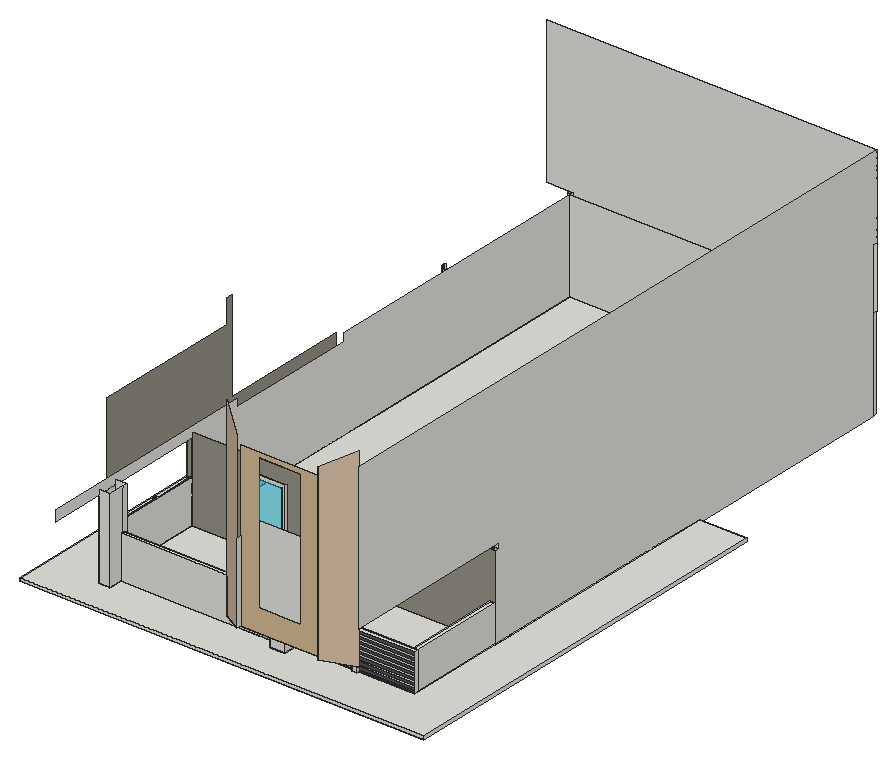
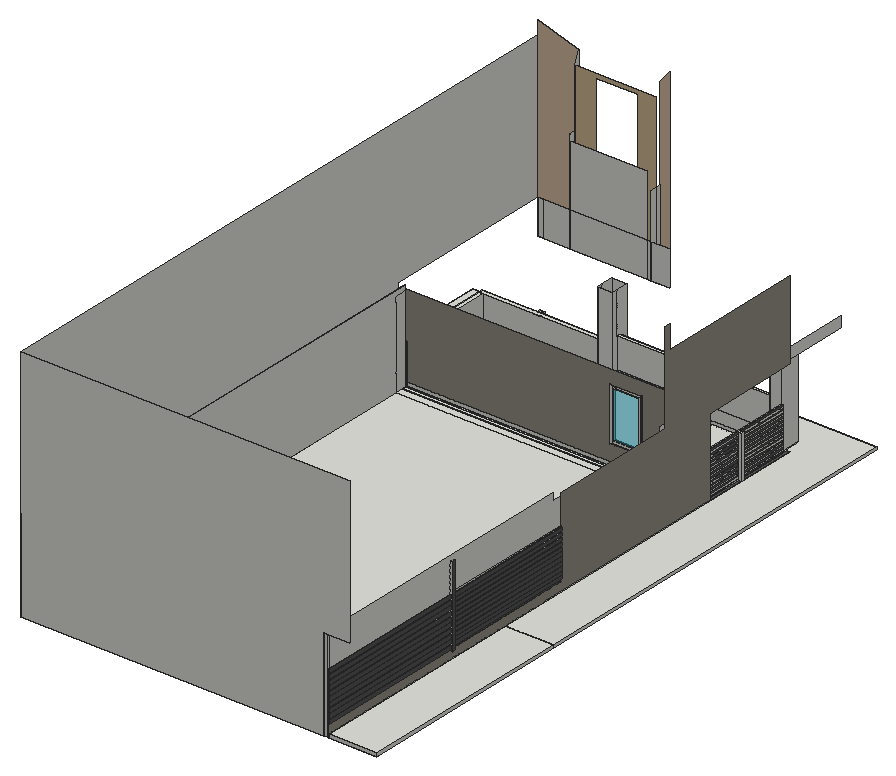
# SketchUp Ruby script. Lengths in inches.
U = 1.inch
M = Sketchup.active_model
def pt(a) = Geom::Point3d.new(a.map { |v| v * U })
def face(e, loops, mat)
  f = e.add_face(loops[0].map { |a| pt(a) })
  loops[1..].each { |l| e.add_face(l.map { |a| pt(a) }).erase! }
  f.material = f.back_material = mat if mat
  f
end
# faces: each face lists its corners as indices into pts; further lists are holes
def faces(e, pts, list, mat = nil) = list.each { |f| face(e, (f[0].is_a?(Array) ? f : [f]).map { |l| l.map { |i| pts[i] } }, mat) }
# xy, xz, yz: faces in a plane at the given z, y or x. An outline is a flat list of corners, or four numbers for a rectangle; further outlines are holes
def ring(l) = l.size == 4 ? [[l[0], l[1]], [l[2], l[1]], [l[2], l[3]], [l[0], l[3]]] : l.each_slice(2).to_a
def flat(e, list, mat, &to3) = list.each { |f| face(e, (f[0].is_a?(Array) ? f : [f]).map { |l| ring(l).map { |u, v| to3.(u, v) } }, mat) }
def xy(e, z, list, mat = nil) = flat(e, list, mat) { |x, y| [x, y, z] }
def xz(e, y, list, mat = nil) = flat(e, list, mat) { |x, z| [x, y, z] }
def yz(e, x, list, mat = nil) = flat(e, list, mat) { |y, z| [x, y, z] }
def lines(e, pts, list) = list.each { |a, b| e.add_line(pt(pts[a]), pt(pts[b])) }
# prism: a flat outline (further loops are holes) pulled along v
def prism(e, loops, v, mat = nil)
  f = face(e, loops, mat); d = Geom::Vector3d.new(v.map { |x| x * U })
  f.pushpull(f.normal.samedirection?(d) ? d.length : -d.length)
end
def box(e, o, s, mat = nil) = prism(e, [[o, [o[0] + s[0], o[1], o[2]], [o[0] + s[0], o[1] + s[1], o[2]], [o[0], o[1] + s[1], o[2]]]], [0, 0, s[2]], mat)
def at(x, y, z, deg = 0) = Geom::Transformation.translation(pt([x, y, z])) * Geom::Transformation.rotation(ORIGIN, Z_AXIS, deg.degrees)
def axes(o, x, y, z) = Geom::Transformation.new([*x, 0, *y, 0, *z, 0, *pt(o).to_a, 1])
def part(name) = M.definitions.add(name)
# library, detail: a bought-in or finely detailed component or shape, given as its bounding box
def library(name, o, s) = part(name).tap { |d| box(d.entities, o, s) }
def detail(e, o, s) = box(e.add_group.entities, o, s)
def put(e, d, t, mat = nil) = e.add_instance(d, t).tap { |i| i.material = mat if mat }
def group(e, t, mat = nil) = e.add_group.tap { |g| g.transformation = t; g.material = mat if mat }.entities
root = M.entities
M.materials.add("[Color M06]").color = [86, 86, 86]
M.materials.add("[Formica Beige]").color = [211, 187, 149]
M.materials.add("[Formica Graystone]").color = [149, 146, 135]
M.materials.add("[Formica Laminate Light]").color = [213, 189, 164]
M.materials.add("[Translucent Glass Tinted]").color = [8, 201, 241]
M.materials["[Translucent Glass Tinted]"].alpha = 0.48
xy(root,0,[[0,101.614,0,889.277,93.831,889.277,93.831,195.446,102.831,195.446,102.831,163.383,125.644,163.383,125.644,195.446,431.545,195.446,431.545,169.758,461.17,169.758,461.17,195.446,693.831,195.446,693.831,391.508,695.081,391.508,695.081,889.277,787.663,889.277,787.663,101.614],[102.831,163.383,125.644,204.446],[93.831,195.446,102.831,391.508],[125.644,195.446,431.545,204.446],[461.17,195.446,461.17,204.446,684.831,204.446,684.831,391.508,693.831,391.508,693.831,195.446],
  [102.831,204.446,684.831,391.508],[93.831,391.508,102.831,400.508],[102.831,391.508,684.831,400.508],[684.831,391.508,693.831,400.508],[693.831,391.508,695.081,400.508],
  [93.831,400.508,102.831,795.446],[102.831,400.508,102.831,406.508,684.831,406.508,684.831,795.446,693.831,795.446,693.831,400.508],[693.831,400.508,695.081,795.446],[102.831,406.508,102.831,795.446,103.706,795.446,103.706,1311.696,684.831,1311.696,684.831,406.508],[93.831,795.446,94.956,889.277],
  [94.956,795.446,102.831,889.277],[102.831,795.446,103.706,889.277],[684.831,795.446,693.831,889.277],[693.831,795.446,695.081,889.277],[0,889.277,93.831,1320.696],
  [93.831,889.277,94.956,1320.696],[94.956,889.277,102.831,1311.696],[102.831,889.277,103.706,1311.696],[684.831,889.277,693.831,1311.696],[693.831,889.277,695.081,1311.696],
  [94.956,1311.696,102.831,1320.696],[102.831,1311.696,103.706,1320.696],[103.706,1311.696,693.831,1320.696]])
xy(root,2,[[94.956,400.508,681.831,406.508],[681.831,400.508,681.894,406.508],[94.956,406.508,102.831,422.071],[102.831,406.508,681.831,422.071],[681.831,406.508,681.894,795.446],
  [681.894,406.508,684.831,795.446],[94.956,422.071,102.831,795.446],[102.831,422.071,681.831,422.071,681.831,1311.696,103.706,1311.696,103.706,795.446,102.831,795.446],[681.831,795.446,681.894,889.277],[681.894,795.446,684.831,889.277],
  [681.831,889.277,681.894,1311.696],[681.894,889.277,684.831,1311.696]])
xy(root,5.187,[[93.706,307.096,99.706,313.624]])
xy(root,6,[[0,101.614,787.663,101.614,787.663,889.277,695.081,889.277,695.081,391.508,693.831,391.508,693.831,195.446,461.17,195.446,461.17,169.758,431.545,169.758,431.545,188.783,125.644,188.783,125.644,163.383,102.831,163.383,102.831,195.446,93.831,195.446,93.831,889.277,0,889.277],[125.644,188.783,431.545,195.446],[99.706,195.446,102.831,204.446],[461.17,195.446,693.831,204.446],[102.831,204.446,684.831,391.508],
  [684.831,204.446,693.831,391.508],[0,889.277,93.831,1320.696]])
xy(root,6,[[93.831,195.446,99.706,391.508]],"[Color M06]")
xy(root,7,[[577.501,189.446,585.653,195.446]])
xy(root,23.1875,[[87.831,1019.031,93.831,1025.522]])
xy(root,24.75,[[90.831,1025.522,93.831,1320.696]])
xy(root,29.206,[[91.331,755.008,93.831,1019.031]])
xy(root,31.875,[[90.831,1025.522,93.831,1311.696],[90.831,1311.696,93.831,1320.696]])
xy(root,34.625,[[90.831,1025.522,93.831,1320.696]])
xy(root,35.1875,[[91.331,755.008,93.831,761.772],[91.331,761.772,93.831,1019.031]])
xy(root,36.893,[[91.331,755.008,93.831,1019.031]])
xy(root,37.873,[[225.269,388.508,287.381,391.508]])
xy(root,41.75,[[90.831,1025.522,93.831,1311.696],[90.831,1311.696,93.831,1320.696]])
xy(root,42.875,[[91.331,755.008,93.831,761.772],[91.331,761.772,93.831,1019.031]])
xy(root,44.5,[[90.831,1025.522,93.831,1320.696]])
xy(root,44.643,[[90.831,755.008,91.331,1019.031],[91.331,755.008,93.831,1019.031]])
xy(root,44.836,[[232.231,388.508,280.419,391.508]])
xy(root,50.625,[[90.831,755.008,91.331,761.772],[91.331,755.008,93.831,761.772],[90.831,761.772,91.331,1019.031],[91.331,761.772,93.831,1019.031]])
xy(root,51.625,[[90.831,1025.522,93.831,1311.696],[90.831,1311.696,93.831,1320.696]])
xy(root,53.268,[[90.831,755.008,93.831,1019.031]])
xy(root,54.375,[[90.831,1025.522,93.831,1320.696]])
xy(root,59.25,[[90.831,755.008,93.831,761.772],[90.831,761.772,93.831,1019.031]])
xy(root,61.5,[[90.831,1025.522,93.831,1311.696],[90.831,1311.696,93.831,1320.696]])
xy(root,61.893,[[90.831,755.008,93.831,1019.031]])
xy(root,64.25,[[90.831,1025.522,93.831,1320.696]])
xy(root,67.875,[[90.831,755.008,93.831,761.772],[90.831,761.772,93.831,1019.031]])
xy(root,70.518,[[90.831,755.008,93.831,1019.031]])
xy(root,71.375,[[90.831,1311.696,93.831,1320.696]])
xy(root,71.375,[[90.831,1025.522,93.831,1311.696]],"[Color M06]")
xy(root,74.125,[[90.831,1025.522,93.831,1320.696],[93.831,1025.522,94.519,1320.696]])
xy(root,76.5,[[90.831,755.008,93.831,761.772],[90.831,761.772,93.831,1019.031]])
xy(root,78,[[577.501,189.446,585.653,195.446],[461.17,195.446,693.831,204.446],[684.831,204.446,693.831,391.508]])
xy(root,79.143,[[90.831,755.008,93.831,1019.031]])
xy(root,81.25,[[90.831,1025.522,93.831,1311.696],[93.831,1025.522,94.519,1311.696],[90.831,1311.696,93.831,1320.696],[93.831,1311.696,94.519,1320.696]])
xy(root,84,[[90.831,1025.522,93.831,1320.696]])
xy(root,85.125,[[90.831,755.008,93.831,761.772],[90.831,761.772,93.831,1019.031]])
xy(root,87.768,[[90.831,755.008,93.831,1019.031]])
xy(root,89.6875,[[99.706,204.446,102.831,204.446,102.831,391.508,99.706,391.508,99.706,313.624,93.706,313.624,93.706,307.096,99.706,307.096]])
xy(root,90,[[125.644,188.783,431.545,195.446]])
xy(root,91.125,[[90.831,1025.522,93.831,1311.696],[90.831,1311.696,93.831,1320.696]])
xy(root,93.75,[[90.831,755.008,93.831,761.772],[90.831,761.772,93.831,1019.031]])
xy(root,93.875,[[90.831,1025.522,93.831,1320.696]])
xy(root,96.393,[[90.831,755.008,93.831,1019.031]])
xy(root,101,[[90.831,1025.522,93.831,1311.696],[90.831,1311.696,93.831,1320.696]])
xy(root,102.375,[[90.831,755.008,93.831,761.772],[90.831,761.772,93.831,1019.031]])
xy(root,103.75,[[90.831,1025.522,93.831,1320.696]])
xy(root,105.018,[[90.831,755.008,93.831,1019.031]])
xy(root,110.875,[[90.831,1025.522,93.831,1311.696],[90.831,1311.696,93.831,1320.696]])
xy(root,111,[[90.831,755.008,93.831,761.772],[90.831,761.772,93.831,1019.031]])
xy(root,111.9375,[[473.833,37.618,436.704,59.368,473.833,59.368],[632.121,37.618,632.121,59.368,693.831,59.368],[473.833,47.368,482.184,59.368],[482.184,47.368,482.184,59.368,632.121,59.113,632.121,47.368]])
xy(root,113.625,[[90.831,1025.522,93.831,1320.696]])
xy(root,113.643,[[90.831,755.008,93.831,1019.031]])
xy(root,119.625,[[90.831,755.008,93.831,761.772],[90.831,761.772,93.831,1019.031]])
xz(root,47.368,[[[473.833,111.9375,632.121,427.928],[509.462,155.324,590.928,419.478]]],"[Formica Beige]")
xz(root,59.368,[[436.704,111.9375,473.833,180],[473.833,111.9375,482.184,180],[482.184,111.9375,632.121,180],[632.121,111.9375,684.831,180],[684.831,111.9375,693.831,180]])
xz(root,101.614,[[0,0,787.663,6]])
xz(root,163.383,[[102.831,0,125.644,6],[102.831,6,125.644,169.522]])
xz(root,169.758,[[431.545,0,461.17,6],[431.545,6,461.17,169.522]])
xz(root,188.783,[[125.644,6,431.545,90]])
xz(root,189.446,[[577.501,7,585.653,78]])
xz(root,195.446,[[93.831,0,102.831,6],[125.644,0,431.545,6],[461.17,0,693.831,1.092],[461.17,1.092,693.831,6],[125.644,6,431.545,30],
  [461.17,6,693.831,7],[461.17,7,577.501,9.967],[577.501,7,585.653,9.967],[577.501,9.967,585.653,15.875],[461.17,15.875,577.501,18.842],
  [577.501,15.875,585.653,18.842],[585.653,15.875,693.831,18.842],[577.501,18.842,585.653,24.75],[461.17,24.75,577.501,27.717],[577.501,24.75,585.653,27.717],
  [585.653,24.75,693.831,27.717],[577.501,27.717,585.653,33.625],[125.644,30,431.545,90],[461.17,33.625,577.501,36.592],[577.501,33.625,585.653,36.592],
  [585.653,33.625,693.831,36.592],[577.501,36.592,585.653,42.5],[461.17,42.5,577.501,45.467],[577.501,42.5,585.653,45.467],[585.653,42.5,693.831,45.467],
  [577.501,45.467,585.653,51.375],[461.17,51.375,577.501,54.342],[577.501,51.375,585.653,54.342],[585.653,51.375,693.831,54.342],[577.501,54.342,585.653,60.25],
  [461.17,60.25,577.501,63.217],[577.501,60.25,585.653,63.217],[585.653,60.25,693.831,63.217],[577.501,63.217,585.653,69.125],[461.17,69.125,577.501,72.092],
  [577.501,69.125,585.653,72.092],[585.653,69.125,693.831,72.092],[577.501,72.092,585.653,78]])
xz(root,195.446,[[585.653,7,693.831,9.967],[461.17,9.967,577.501,15.875],[585.653,9.967,693.831,15.875],[461.17,18.842,577.501,24.75],[585.653,18.842,693.831,24.75],
  [461.17,27.717,577.501,33.625],[585.653,27.717,693.831,33.625],[461.17,36.592,577.501,42.5],[585.653,36.592,693.831,42.5],[461.17,45.467,577.501,51.375],
  [585.653,45.467,693.831,51.375],[461.17,54.342,577.501,60.25],[585.653,54.342,693.831,60.25],[461.17,63.217,577.501,69.125],[585.653,63.217,693.831,69.125],
  [461.17,72.092,577.501,78],[585.653,72.092,693.831,78]],"[Color M06]")
xz(root,204.446,[[102.831,0,125.644,6],[125.644,0,431.545,6],[431.545,0,461.17,6],[461.17,0,684.831,6],[99.706,6,102.831,89.6875],
  [102.831,6,125.644,169.522],[431.545,6,461.17,169.522],[461.17,6,684.831,78],[684.831,6,693.831,78]])
xz(root,307.096,[[93.706,5.187,99.706,89.6875]])
xz(root,313.624,[[93.706,5.187,99.706,89.6875]])
xz(root,388.508,[[[225.269,37.873,287.381,142.674],[232.231,44.836,280.419,135.711]]])
xz(root,391.508,[[93.831,0,102.831,0,102.831,89.6875,99.706,89.6875,99.706,6,93.831,6],[102.831,0,684.831,6],[684.831,0,693.831,6],[693.831,0,695.081,6],[93.831,6,99.706,89.6875],
  [684.831,6,693.831,78]])
xz(root,391.508,[[[102.831,6,684.831,6,684.831,78,693.831,78,693.831,6,695.081,6,695.081,169.522,102.831,169.522],[225.269,37.873,287.381,142.674]],[93.831,89.6875,102.831,158.522]],"[Formica Graystone]")
xz(root,391.508,[[232.231,44.836,280.419,135.711]],"[Translucent Glass Tinted]")
xz(root,400.508,[[693.831,0,695.081,2],[681.831,2,681.894,169.522],[681.894,2,684.519,169.522],[684.519,2,684.831,169.522],[684.831,2,693.831,169.522]])
xz(root,406.508,[[102.831,0,684.831,2]])
xz(root,755.008,[[91.331,29.206,93.831,35.1875],[91.331,36.893,93.831,42.875],[90.831,44.643,91.331,50.625],[91.331,44.643,93.831,50.625],[90.831,53.268,93.831,59.25],
  [90.831,61.893,93.831,67.875],[90.831,70.518,93.831,76.5],[90.831,79.143,93.831,85.125],[90.831,87.768,93.831,93.75],[90.831,96.393,93.831,102.375],
  [90.831,105.018,93.831,111],[90.831,113.643,93.831,119.625]])
xz(root,795.446,[[94.956,0,102.831,2],[102.831,0,103.706,2]])
xz(root,889.277,[[0,0,93.831,6],[695.081,0,787.663,6]])
xz(root,1019.031,[[87.831,23.1875,93.831,23.1875,93.831,29.206,91.331,29.206,91.331,35.1875,93.831,35.1875,93.831,36.893,91.331,36.893,91.331,42.875,93.831,42.875,93.831,44.643,90.831,44.643,90.831,50.625,93.831,50.625,93.831,53.268,90.831,53.268,90.831,59.25,93.831,59.25,93.831,61.893,90.831,61.893,90.831,67.875,93.831,67.875,93.831,70.518,90.831,70.518,90.831,76.5,93.831,76.5,93.831,79.143,90.831,79.143,90.831,85.125,93.831,85.125,93.831,87.768,90.831,87.768,90.831,93.75,93.831,93.75,93.831,96.393,90.831,96.393,90.831,102.375,93.831,102.375,93.831,105.018,90.831,105.018,90.831,111,93.831,111,93.831,113.643,90.831,113.643,90.831,119.625,93.831,119.625,93.831,122.268,90.831,122.268,90.831,128.25,93.831,128.25,93.831,130.893,90.831,130.893,90.831,136.875,93.831,136.875,93.831,139.518,90.831,139.518,90.831,145.5,93.831,145.5,93.831,148.143,90.831,148.143,90.831,154.125,93.831,154.125,93.831,156.768,90.831,156.768,90.831,162.75,93.831,162.75,93.831,165.393,90.831,165.393,90.831,171.375,93.831,171.375,93.831,174.018,90.831,174.018,90.831,180,87.831,180],[91.331,29.206,93.831,35.1875],[91.331,36.893,93.831,42.875],[90.831,44.643,91.331,50.625],[91.331,44.643,93.831,50.625],
  [90.831,53.268,93.831,59.25],[90.831,61.893,93.831,67.875],[90.831,70.518,93.831,76.5],[90.831,79.143,93.831,85.125],[90.831,87.768,93.831,93.75],
  [90.831,96.393,93.831,102.375],[90.831,105.018,93.831,111],[90.831,113.643,93.831,119.625]])
xz(root,1025.522,[[87.831,23.1875,87.831,180,90.831,180,90.831,172.875,93.831,172.875,93.831,170.125,90.831,170.125,90.831,163,93.831,163,93.831,160.25,90.831,160.25,90.831,153.125,93.831,153.125,93.831,150.375,90.831,150.375,90.831,143.25,93.831,143.25,93.831,140.5,90.831,140.5,90.831,133.375,93.831,133.375,93.831,130.625,90.831,130.625,90.831,123.5,93.831,123.5,93.831,120.75,90.831,120.75,90.831,113.625,93.831,113.625,93.831,110.875,90.831,110.875,90.831,103.75,93.831,103.75,93.831,101,90.831,101,90.831,93.875,93.831,93.875,93.831,91.125,90.831,91.125,90.831,84,93.831,84,93.831,81.25,90.831,81.25,90.831,74.125,93.831,74.125,93.831,71.375,90.831,71.375,90.831,64.25,93.831,64.25,93.831,61.5,90.831,61.5,90.831,54.375,93.831,54.375,93.831,51.625,90.831,51.625,90.831,44.5,93.831,44.5,93.831,41.75,90.831,41.75,90.831,34.625,93.831,34.625,93.831,31.875,90.831,31.875,90.831,24.75,93.831,24.75,93.831,23.1875],[90.831,24.75,93.831,31.875],[90.831,34.625,93.831,41.75],[90.831,44.5,93.831,51.625],[90.831,54.375,93.831,61.5],
  [90.831,64.25,93.831,71.375],[90.831,74.125,93.831,81.25],[93.831,74.125,94.519,81.25],[90.831,84,93.831,91.125],[90.831,93.875,93.831,101],
  [90.831,103.75,93.831,110.875],[90.831,113.625,93.831,120.75]])
xz(root,1311.696,[[94.956,0,103.706,2],[684.831,0,693.831,0,693.831,180,681.894,180,681.894,2,684.831,2],[693.831,0,695.081,180],[103.706,2,681.831,180],[681.831,2,681.894,180]])
xz(root,1320.696,[[0,0,93.831,6],[102.831,0,102.831,180,51.644,180,51.644,463.1875,695.081,463.1875,695.081,180,693.831,180,693.831,0],[93.831,0,93.831,74.125,94.519,74.125,94.519,81.25,93.831,81.25,93.831,180,94.956,180,94.956,0],[94.956,0,102.831,180],[90.831,24.75,93.831,31.875],
  [90.831,34.625,93.831,41.75],[90.831,44.5,93.831,51.625],[90.831,54.375,93.831,61.5],[90.831,64.25,93.831,71.375],[90.831,74.125,93.831,81.25],
  [93.831,74.125,94.519,81.25],[90.831,84,93.831,91.125],[90.831,93.875,93.831,101],[90.831,103.75,93.831,110.875],[90.831,113.625,93.831,120.75]])
yz(root,0,[[101.614,0,889.277,6],[889.277,0,1320.696,6]])
yz(root,87.831,[[1019.031,23.1875,1025.522,180]],"[Color M06]")
yz(root,90.831,[[1025.522,24.75,1320.696,31.875],[1025.522,34.625,1320.696,41.75],[1025.522,44.5,1320.696,51.625],[755.008,44.643,1019.031,50.625],[755.008,53.268,1019.031,59.25],
  [1025.522,54.375,1320.696,61.5],[755.008,61.893,1019.031,67.875],[1025.522,64.25,1320.696,71.375],[755.008,70.518,1019.031,76.5],[1025.522,74.125,1320.696,81.25],
  [755.008,79.143,1019.031,85.125],[1025.522,84,1320.696,91.125],[755.008,87.768,1019.031,93.75],[1025.522,93.875,1320.696,101],[755.008,96.393,1019.031,102.375],
  [1025.522,103.75,1320.696,110.875],[755.008,105.018,1019.031,111],[1025.522,113.625,1320.696,120.75],[755.008,113.643,1019.031,119.625]],"[Color M06]")
yz(root,91.331,[[755.008,44.643,1019.031,50.625]])
yz(root,91.331,[[755.008,29.206,1019.031,35.1875],[755.008,36.893,1019.031,42.875]],"[Color M06]")
yz(root,93.706,[[307.096,5.187,313.624,89.6875]])
yz(root,93.831,[[195.446,0,391.508,6],[391.508,0,400.508,6],[400.508,0,795.446,6],[795.446,0,889.277,6],[889.277,0,1320.696,6],
  [755.008,23.081,1019.031,23.1875],[1025.522,23.1875,1320.696,24.75],[1025.522,24.75,1320.696,31.875],[755.008,29.0625,1019.031,29.206],[755.008,29.206,1019.031,35.1875],
  [1025.522,31.875,1320.696,34.625],[1025.522,34.625,1320.696,41.75],[755.008,35.1875,1019.031,36.893],[755.008,36.893,1019.031,42.875],[1025.522,41.75,1320.696,44.5],
  [755.008,42.875,1019.031,44.643],[1025.522,44.5,1320.696,51.625],[755.008,44.643,1019.031,50.625],[755.008,50.625,1019.031,53.268],[1025.522,51.625,1320.696,54.375],
  [755.008,53.268,1019.031,59.25],[1025.522,54.375,1320.696,61.5],[755.008,59.25,1019.031,61.893],[1025.522,61.5,1320.696,64.25],[755.008,61.893,1019.031,67.875],
  [1025.522,64.25,1320.696,71.375],[755.008,70.518,1019.031,76.5],[1025.522,71.375,1320.696,74.125],[1025.522,74.125,1320.696,81.25],[755.008,76.5,1019.031,79.143],
  [755.008,79.143,1019.031,85.125],[1025.522,81.25,1320.696,84],[1025.522,84,1320.696,91.125],[755.008,87.768,1019.031,93.75],[1025.522,91.125,1320.696,93.875],
  [755.008,93.75,1019.031,96.393],[1025.522,93.875,1320.696,101],[755.008,96.393,1019.031,102.375],[1025.522,101,1320.696,103.75],[755.008,102.375,1019.031,105.018],
  [1025.522,103.75,1320.696,110.875],[755.008,105.018,1019.031,111],[1025.522,110.875,1320.696,113.625],[755.008,111,1019.031,113.643],[1025.522,113.625,1320.696,120.75],
  [755.008,113.643,1019.031,119.625],[755.008,119.625,1019.031,122.268]])
yz(root,93.831,[[755.008,23.1875,1019.031,29.0625],[755.008,67.875,1019.031,70.518],[755.008,85.125,1019.031,87.768]],"[Color M06]")
yz(root,93.831,[[391.508,6,391.508,158.522,194.662,158.522,194.662,312,488.084,312,488.084,358.375,499.931,358.375,499.931,180,755.008,180,755.008,23.081,1019.031,23.081,1019.031,23.1875,1320.696,23.1875,1320.696,6]],"[Formica Graystone]")
yz(root,94.519,[[1025.522,74.125,1320.696,81.25]])
yz(root,99.706,[[204.446,4.124,204.446,6,307.096,6,307.096,5.187,313.624,5.187,313.624,6,391.508,6,391.508,4.124],[307.096,5.187,313.624,6],[307.096,6,313.624,8.6875],[204.446,8.6875,307.096,10.874],[307.096,8.6875,313.624,10.874],
  [313.624,8.6875,391.508,10.874],[307.096,10.874,313.624,15.4375],[307.096,10.874,313.624,69.4375],[204.446,15.4375,307.096,17.624],[307.096,15.4375,313.624,17.624],
  [313.624,15.4375,391.508,17.624],[307.096,17.624,313.624,22.1875],[204.446,22.1875,307.096,24.374],[307.096,22.1875,313.624,24.374],[313.624,22.1875,391.508,24.374],
  [307.096,24.374,313.624,28.9375],[204.446,28.9375,307.096,31.124],[307.096,28.9375,313.624,31.124],[313.624,28.9375,391.508,31.124],[307.096,31.124,313.624,35.6875],
  [204.446,35.6875,307.096,37.874],[307.096,35.6875,313.624,37.874],[313.624,35.6875,391.508,37.874],[307.096,37.874,313.624,42.4375],[204.446,42.4375,307.096,44.624],
  [307.096,42.4375,313.624,44.624],[313.624,42.4375,391.508,44.624],[307.096,44.624,313.624,49.1875],[204.446,49.1875,307.096,51.374],[307.096,49.1875,313.624,51.374],
  [313.624,49.1875,391.508,51.374],[307.096,51.374,313.624,55.9375],[204.446,55.9375,307.096,58.124],[307.096,55.9375,313.624,58.124],[313.624,55.9375,391.508,58.124],
  [307.096,58.124,313.624,62.6875],[204.446,62.6875,307.096,64.874],[307.096,62.6875,313.624,64.874],[313.624,62.6875,391.508,64.874],[307.096,64.874,313.624,69.4375],
  [204.446,69.4375,307.096,71.624],[307.096,69.4375,313.624,71.624],[313.624,69.4375,391.508,71.624],[307.096,71.624,313.624,76.1875],[204.446,76.1875,307.096,78.374],
  [307.096,76.1875,313.624,78.374],[313.624,76.1875,391.508,78.374],[307.096,78.374,313.624,82.9375],[204.446,82.9375,307.096,85.124],[307.096,82.9375,313.624,85.124],
  [313.624,82.9375,391.508,85.124]])
yz(root,99.706,[[204.446,6,307.096,8.6875],[313.624,6,391.508,8.6875],[204.446,10.874,307.096,15.4375],[313.624,10.874,391.508,15.4375],[204.446,17.624,307.096,22.1875],
  [313.624,17.624,391.508,22.1875],[204.446,24.374,307.096,28.9375],[313.624,24.374,391.508,28.9375],[204.446,31.124,307.096,35.6875],[313.624,31.124,391.508,35.6875],
  [204.446,37.874,307.096,42.4375],[313.624,37.874,391.508,42.4375],[204.446,44.624,307.096,49.1875],[313.624,44.624,391.508,49.1875],[204.446,51.374,307.096,55.9375],
  [313.624,51.374,391.508,55.9375],[204.446,58.124,307.096,62.6875],[313.624,58.124,391.508,62.6875],[204.446,64.874,307.096,69.4375],[313.624,64.874,391.508,69.4375],
  [204.446,71.624,307.096,76.1875],[313.624,71.624,391.508,76.1875],[204.446,78.374,307.096,82.9375],[313.624,78.374,391.508,82.9375],[204.446,85.124,307.096,89.6875],
  [313.624,85.124,391.508,89.6875]],"[Color M06]")
yz(root,102.831,[[391.508,0,406.508,0,406.508,2,795.446,2,795.446,0,1320.696,0,1320.696,180,761.772,180,761.772,165,501.147,165,501.147,180,59.446,180,59.446,158.522,391.508,158.522],[163.383,0,195.446,6],[195.446,0,204.446,6],[204.446,0,391.508,6],[406.508,0,795.446,2],
  [163.383,6,204.446,158.522],[204.446,6,391.508,89.6875]])
yz(root,103.706,[[795.446,0,889.277,2],[889.277,0,1311.696,2]])
yz(root,125.644,[[163.383,0,195.446,6],[195.446,0,204.446,169.522],[163.383,6,188.783,6,188.783,90,195.446,90,195.446,169.522,163.383,169.522],[188.783,6,195.446,30],[188.783,30,195.446,90]])
yz(root,225.269,[[388.508,37.873,391.508,142.674]])
yz(root,232.231,[[388.508,44.836,391.508,135.711]])
yz(root,280.419,[[388.508,44.836,391.508,135.711]])
yz(root,287.381,[[388.508,37.873,391.508,142.674]])
yz(root,431.545,[[169.758,0,195.446,6],[195.446,0,204.446,169.522],[169.758,6,169.758,169.522,195.446,169.522,195.446,90,188.783,90,188.783,6],[188.783,6,195.446,30],[188.783,30,195.446,90]])
yz(root,461.17,[[169.758,0,195.446,6],[195.446,0,204.446,6],[169.758,6,195.446,169.522],[195.446,6,204.446,78],[195.446,78,204.446,169.522]])
yz(root,473.833,[[37.618,111.9375,47.368,269.226],[47.368,111.9375,59.368,269.226]])
yz(root,577.501,[[189.446,7,195.446,78]])
yz(root,585.653,[[189.446,7,195.446,78]])
yz(root,632.121,[[37.618,111.9375,37.618,450.147,47.368,427.928,47.368,111.9375],[47.368,111.9375,59.113,312],[59.113,111.9375,59.368,312]])
yz(root,681.831,[[400.508,2,422.071,169.522],[422.071,2,422.071,169.522,400.508,169.522,400.508,180,1311.696,180,1311.696,2]])
yz(root,681.894,[[400.508,2,1311.696,180]])
yz(root,684.831,[[204.446,0,391.508,6],[406.508,0,795.446,2],[795.446,0,889.277,2],[889.277,0,1311.696,2],[204.446,6,391.508,78]])
yz(root,693.831,[[195.446,0,391.508,6],[1311.696,0,1320.696,180],[195.446,6,204.446,78],[204.446,6,391.508,78]])
yz(root,695.081,[[889.277,0,1311.696,0,1311.696,300,1320.696,300,1320.696,463.1875,59.368,463.1875,59.368,180,400.508,180,400.508,169.522,391.508,169.522,391.508,6,889.277,6],[391.508,0,400.508,2],[400.508,0,795.446,6],[795.446,0,889.277,6],[391.508,2,400.508,6]])
yz(root,787.663,[[101.614,0,889.277,6]])
p = [[573.001,204.446,78],[573.001,195.446,7],[577.501,195.446,7],[585.653,195.446,7],[585.653,204.446,78],[473.833,37.618,269.226],
  [473.833,37.618,450.147],[436.704,59.368,489.375],[436.704,59.368,300],[436.704,59.368,299.8125],[436.704,59.368,180],[436.704,59.368,111.9375],
  [473.833,37.618,111.9375],[693.831,59.368,300],[693.831,59.368,358.375],[693.831,59.368,463.1875],[693.831,59.368,489.375],[632.121,37.618,450.147],
  [632.121,37.618,111.9375],[693.831,59.368,111.9375],[693.831,59.368,180],[482.184,59.368,299.8125],[482.184,59.368,300],[632.121,59.113,300],
  [632.121,59.113,111.9375],[482.184,59.368,111.9375],[482.184,59.368,180],[103.706,1320.696,120],[102.831,1320.696,120],[94.956,400.508,2],
  [93.831,400.508,2],[94.956,391.508,2],[693.831,400.508,2],[693.831,391.508,2],[99.706,391.508,1.9375],[99.706,204.446,1.9375],
  [99.706,391.508,0]]
faces(root,p,[[0,1,2,3,4],[21,22,23,24,25,26]])
faces(root,p,[[5,6,7,8,9,10,11,12],[13,14,15,16,17,18,19,20]],"[Formica Laminate Light]")
lines(root,p,[[27,28],[29,30],[29,31],[32,33],[34,35],[36,34]])
